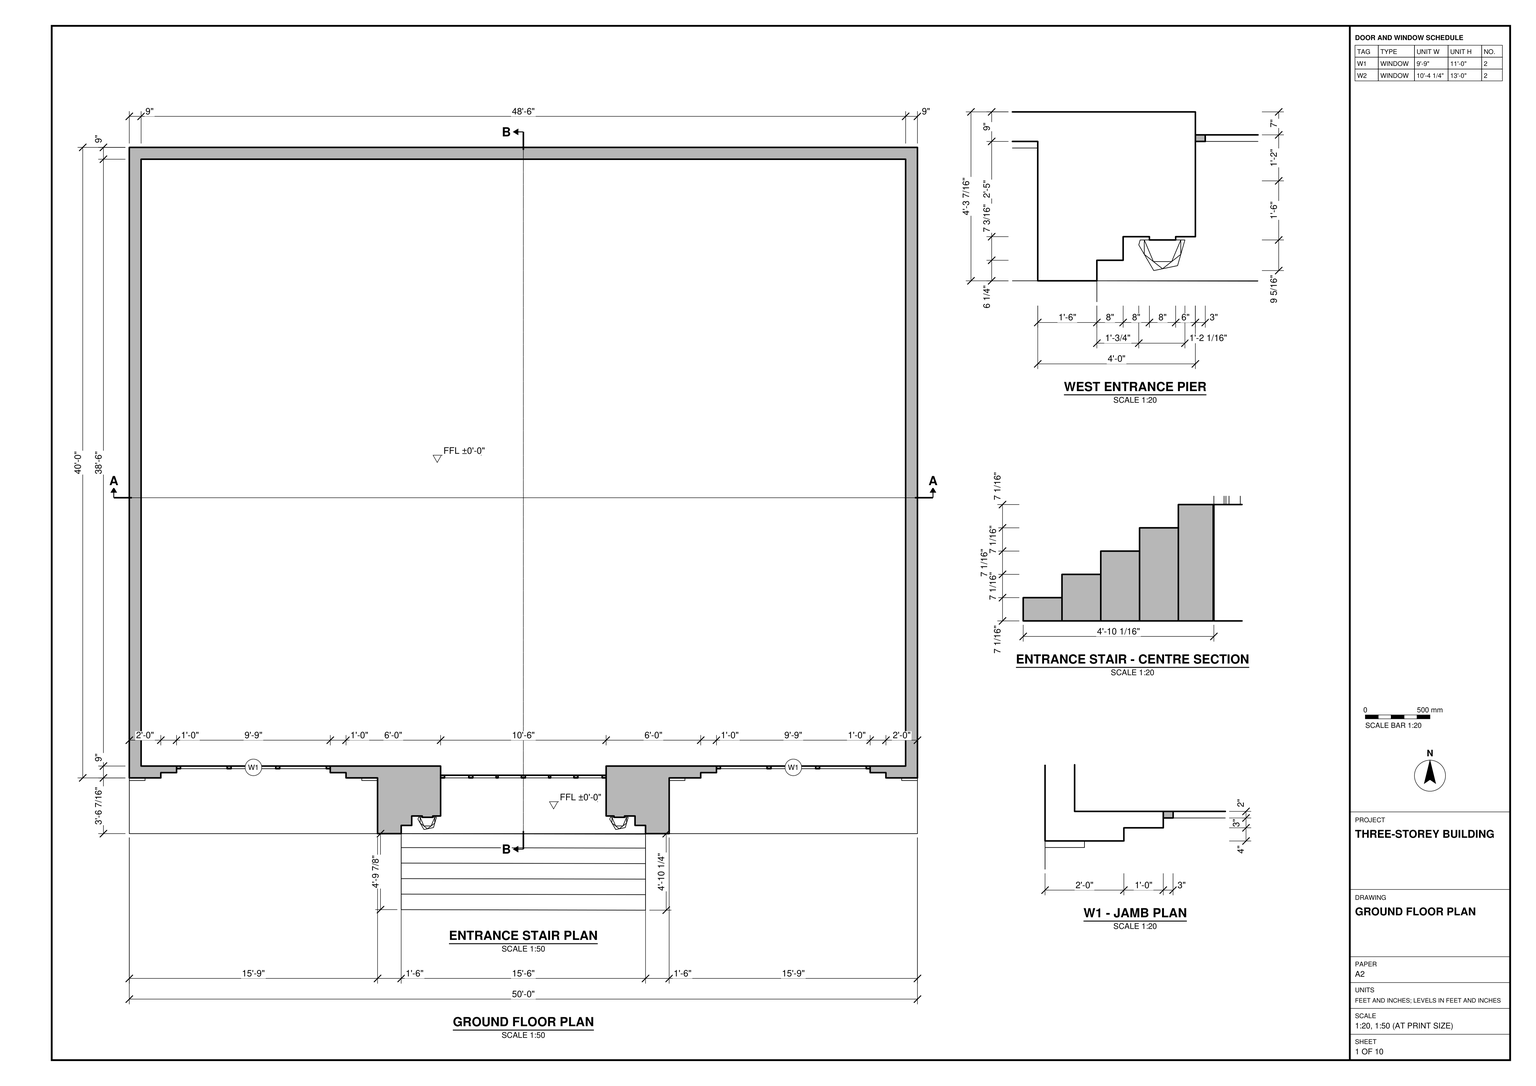
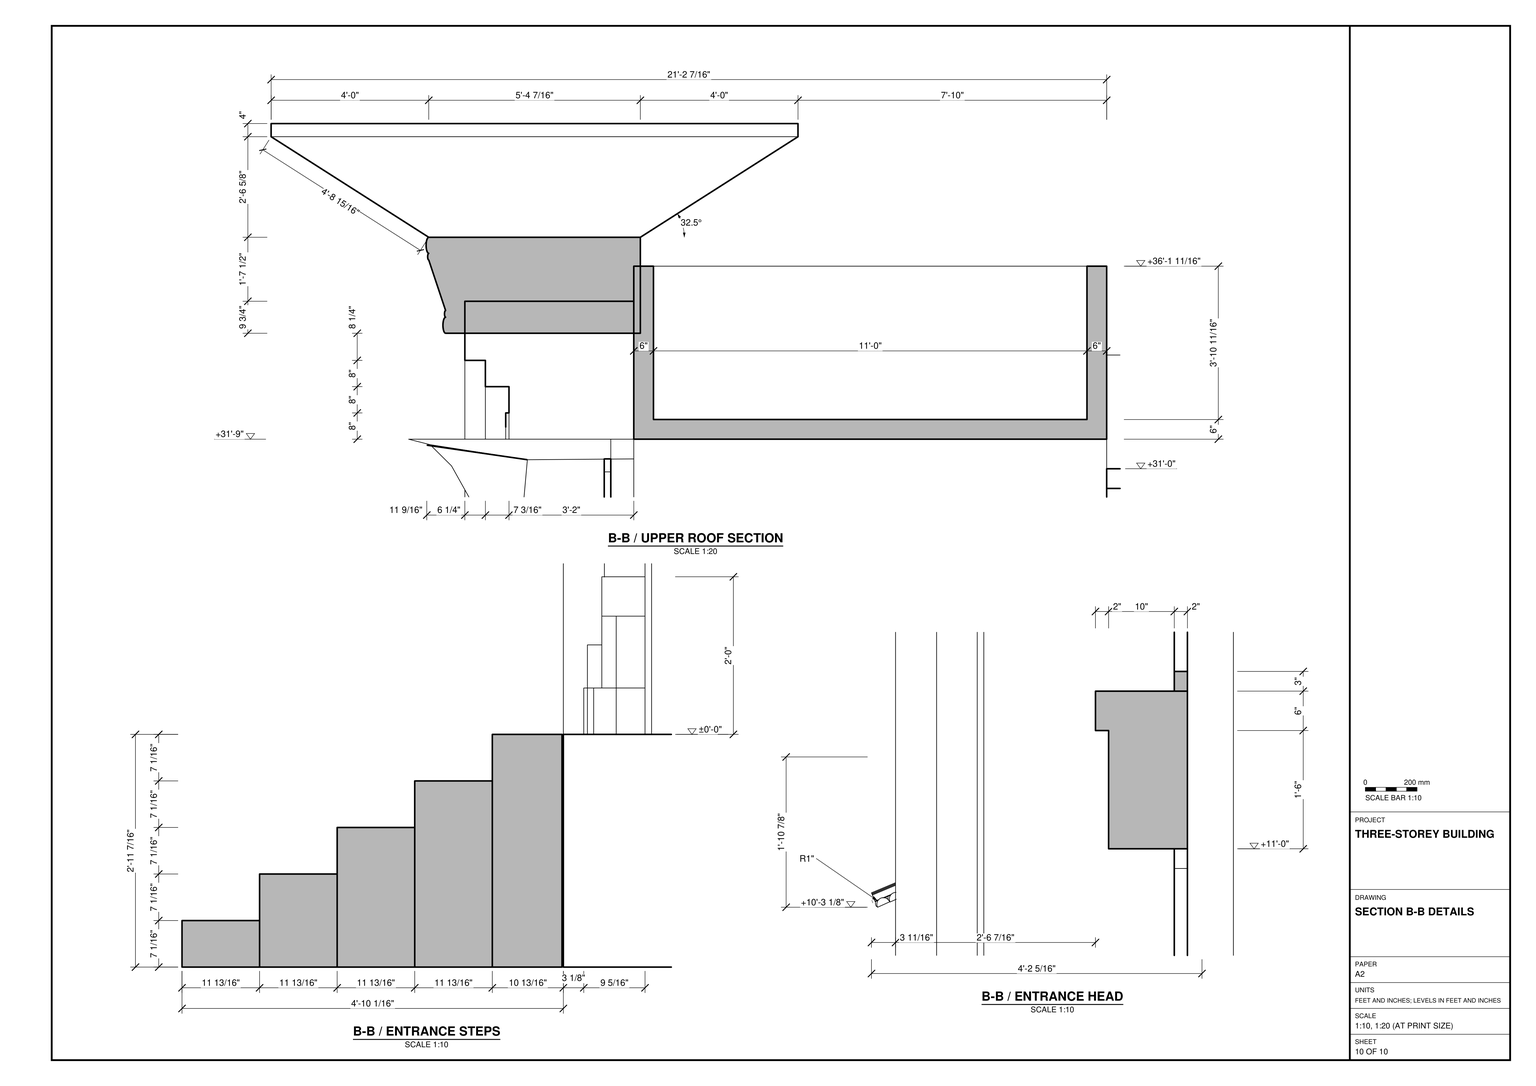
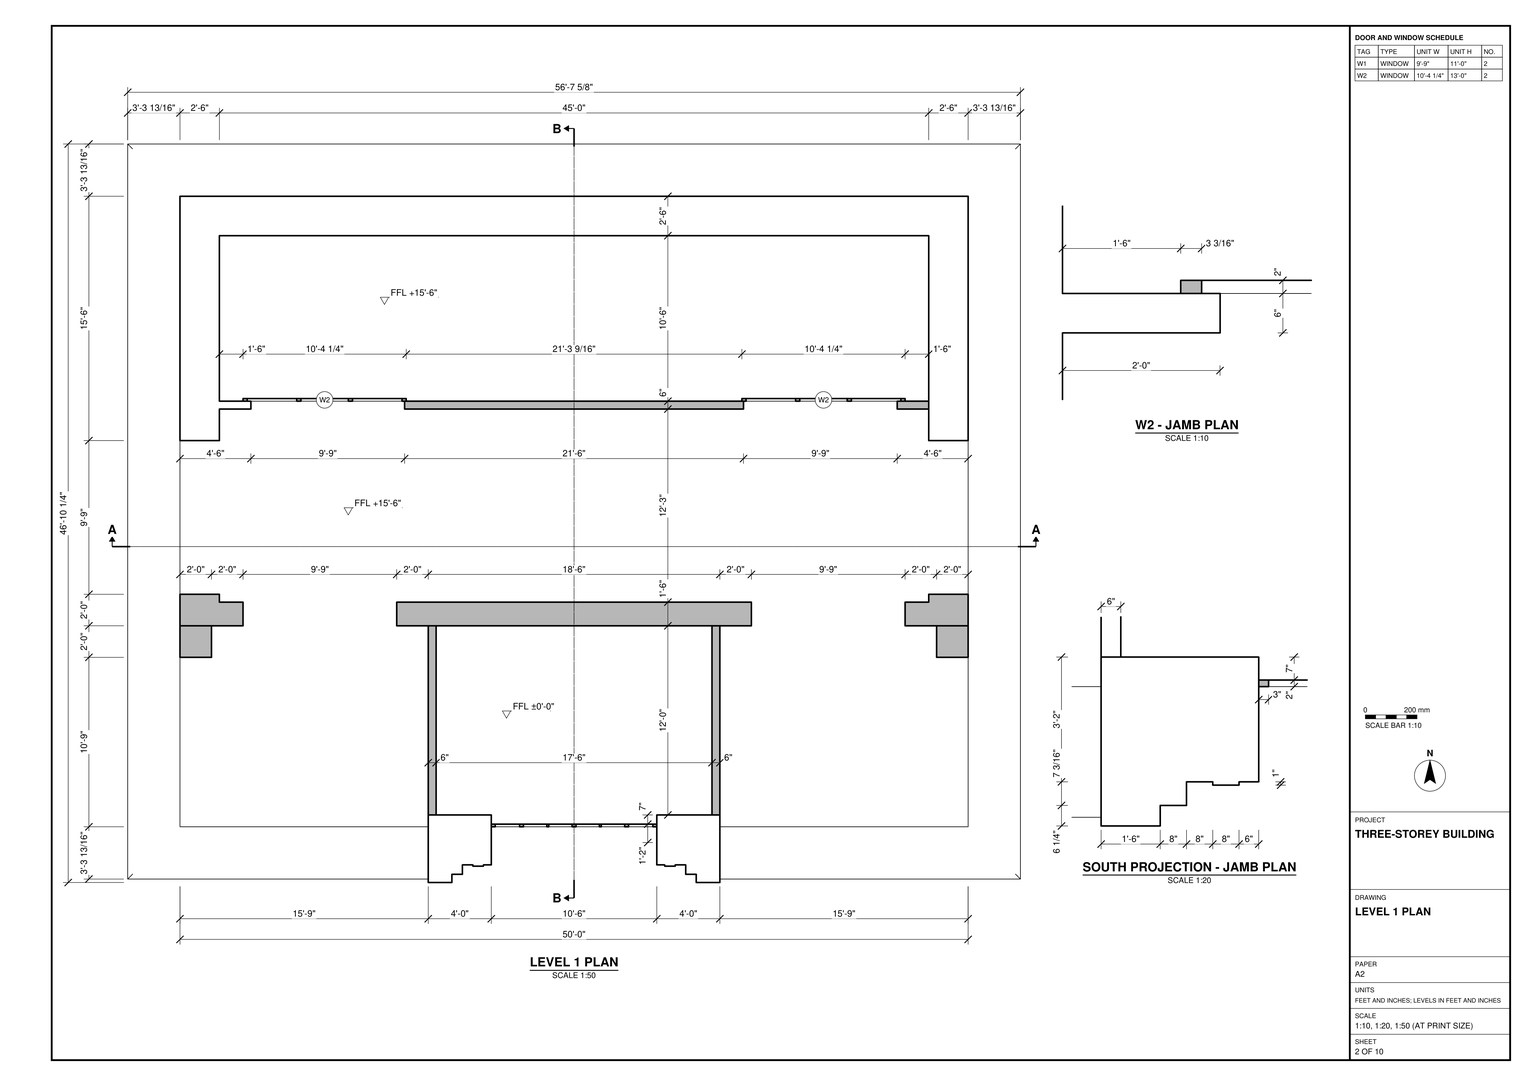
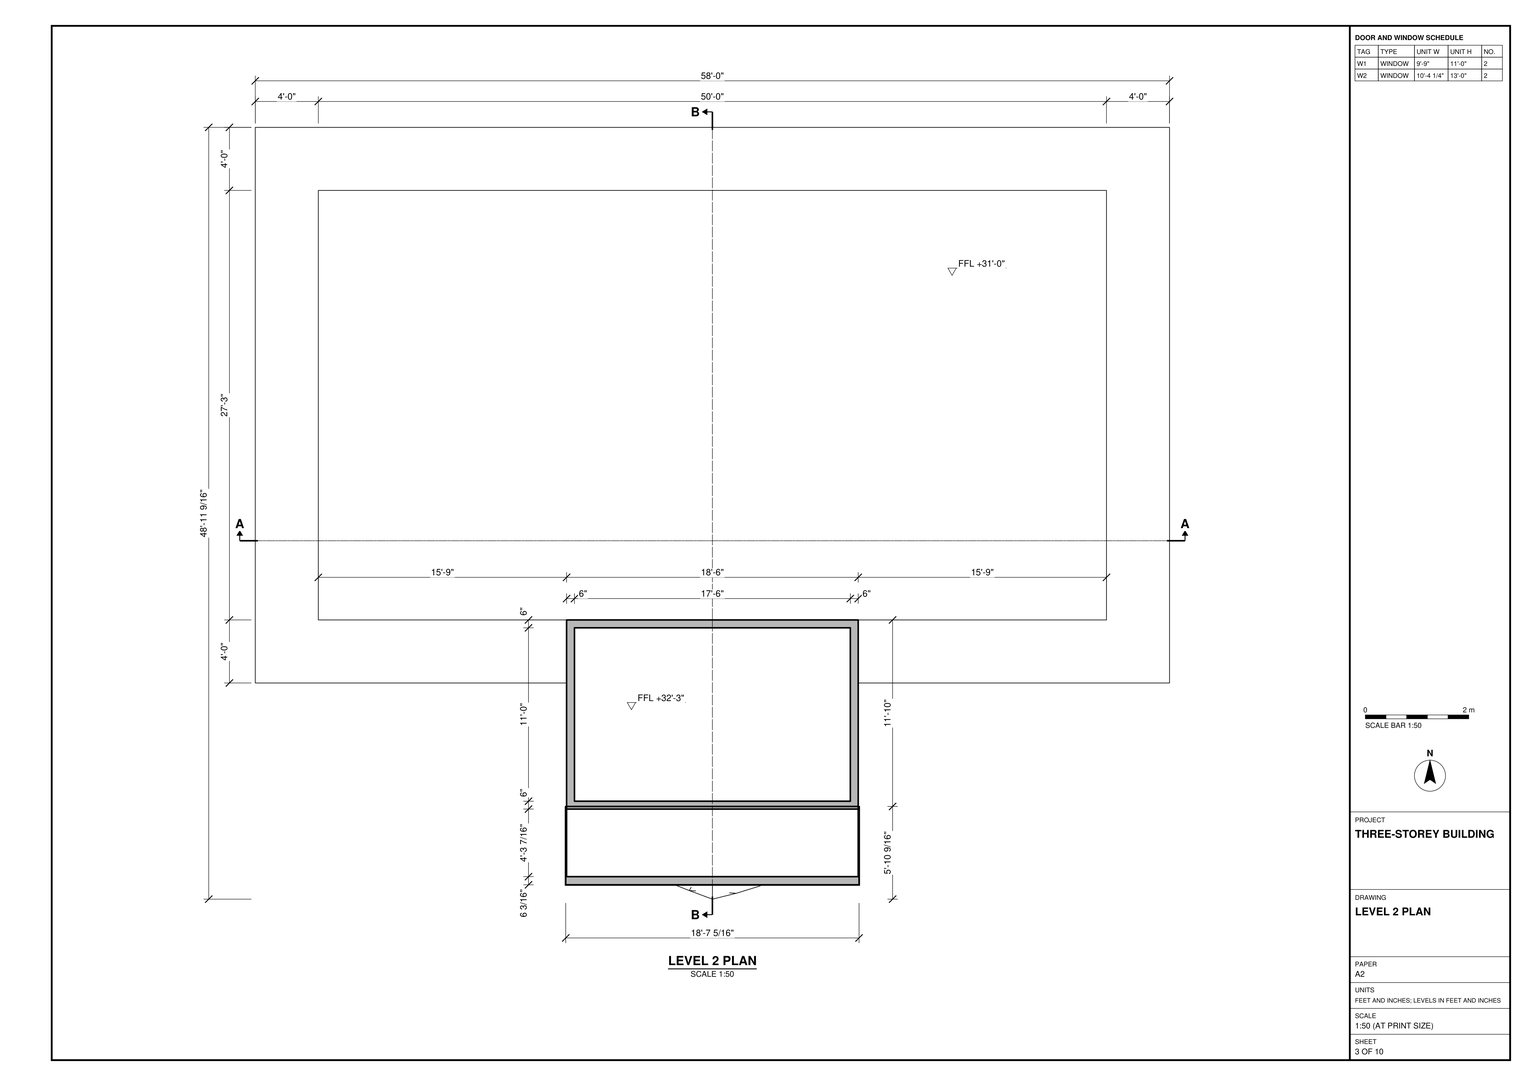
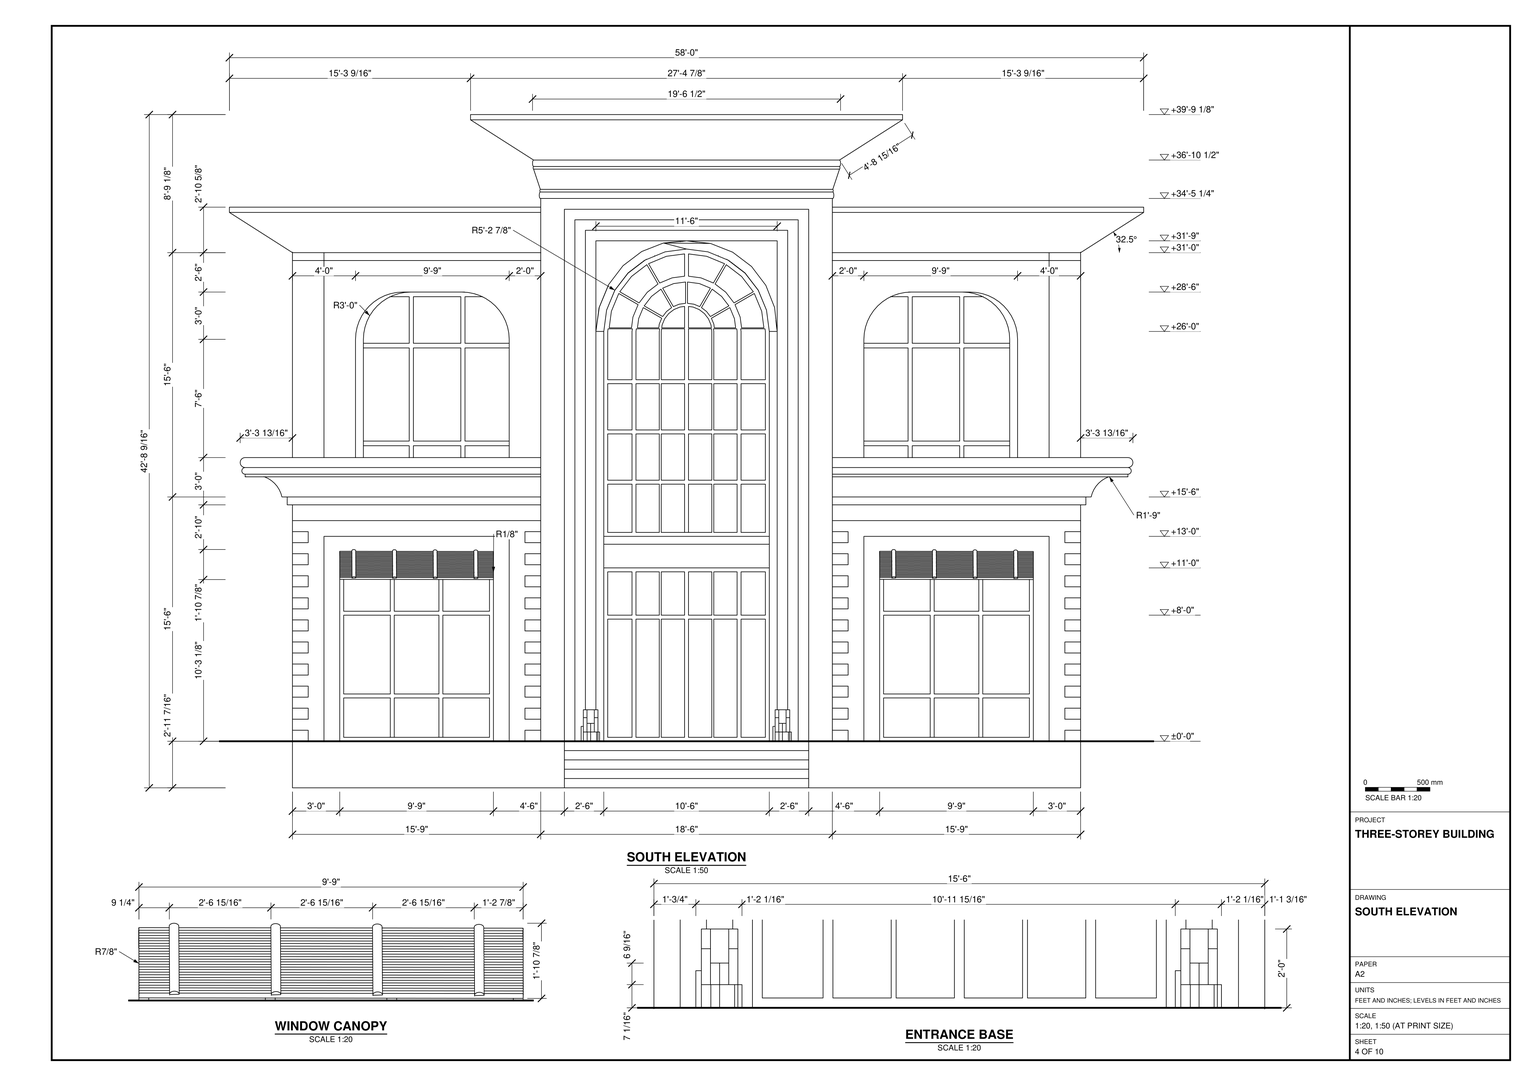
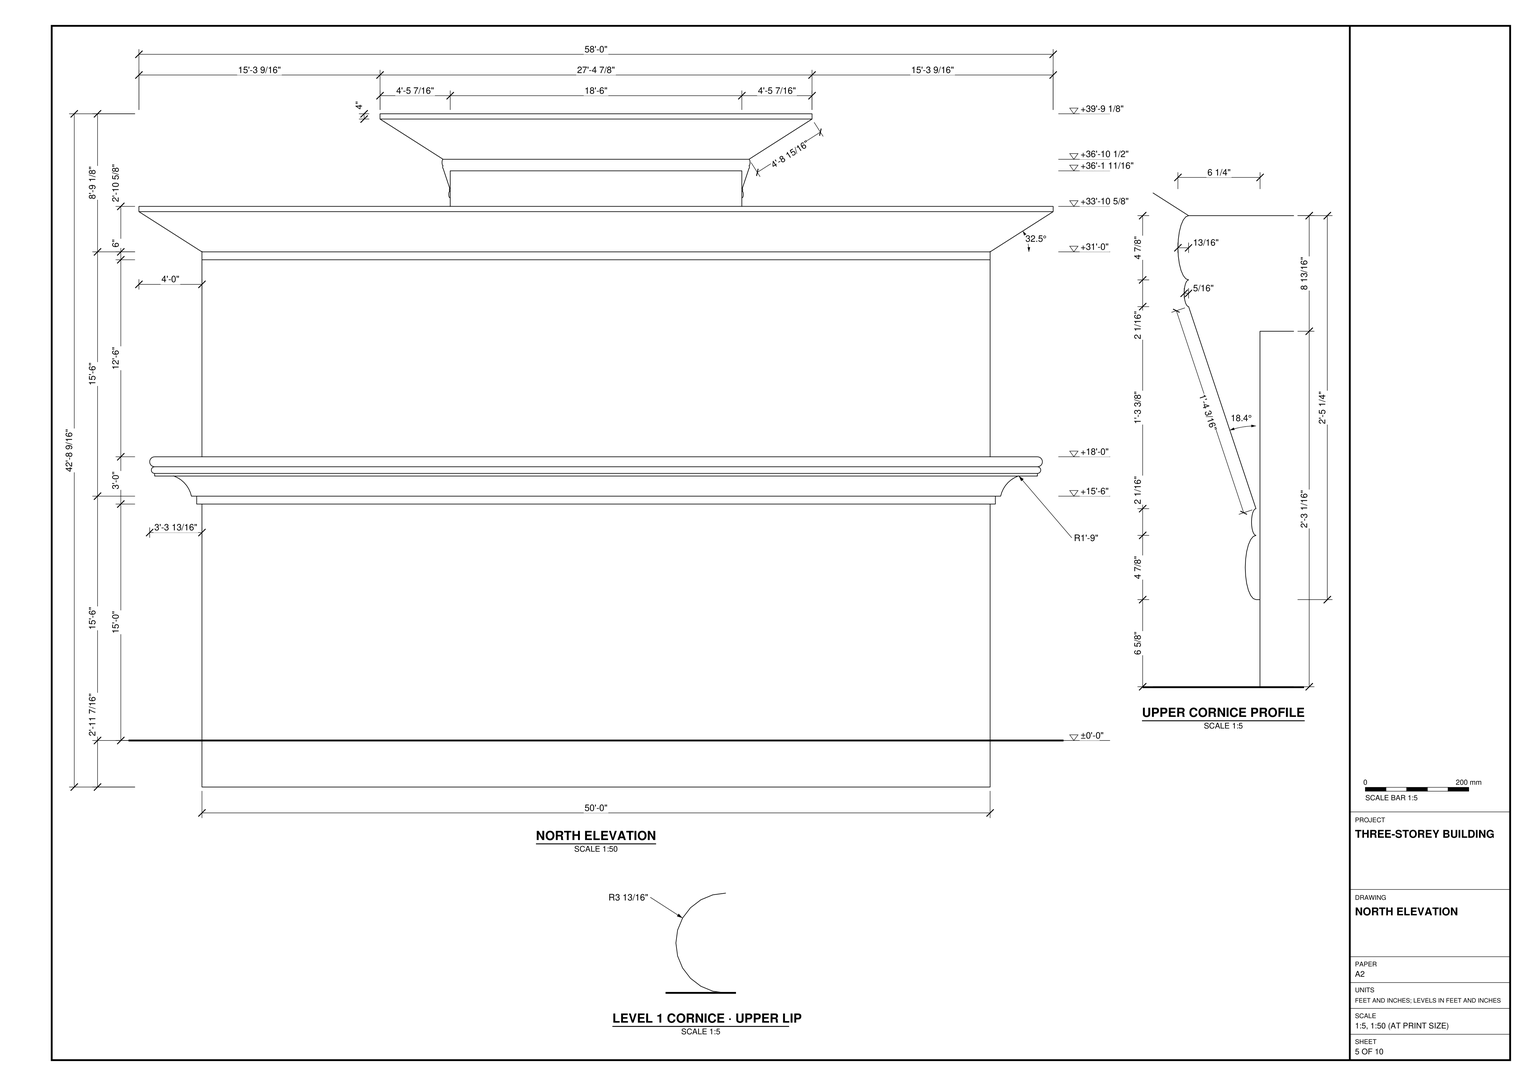
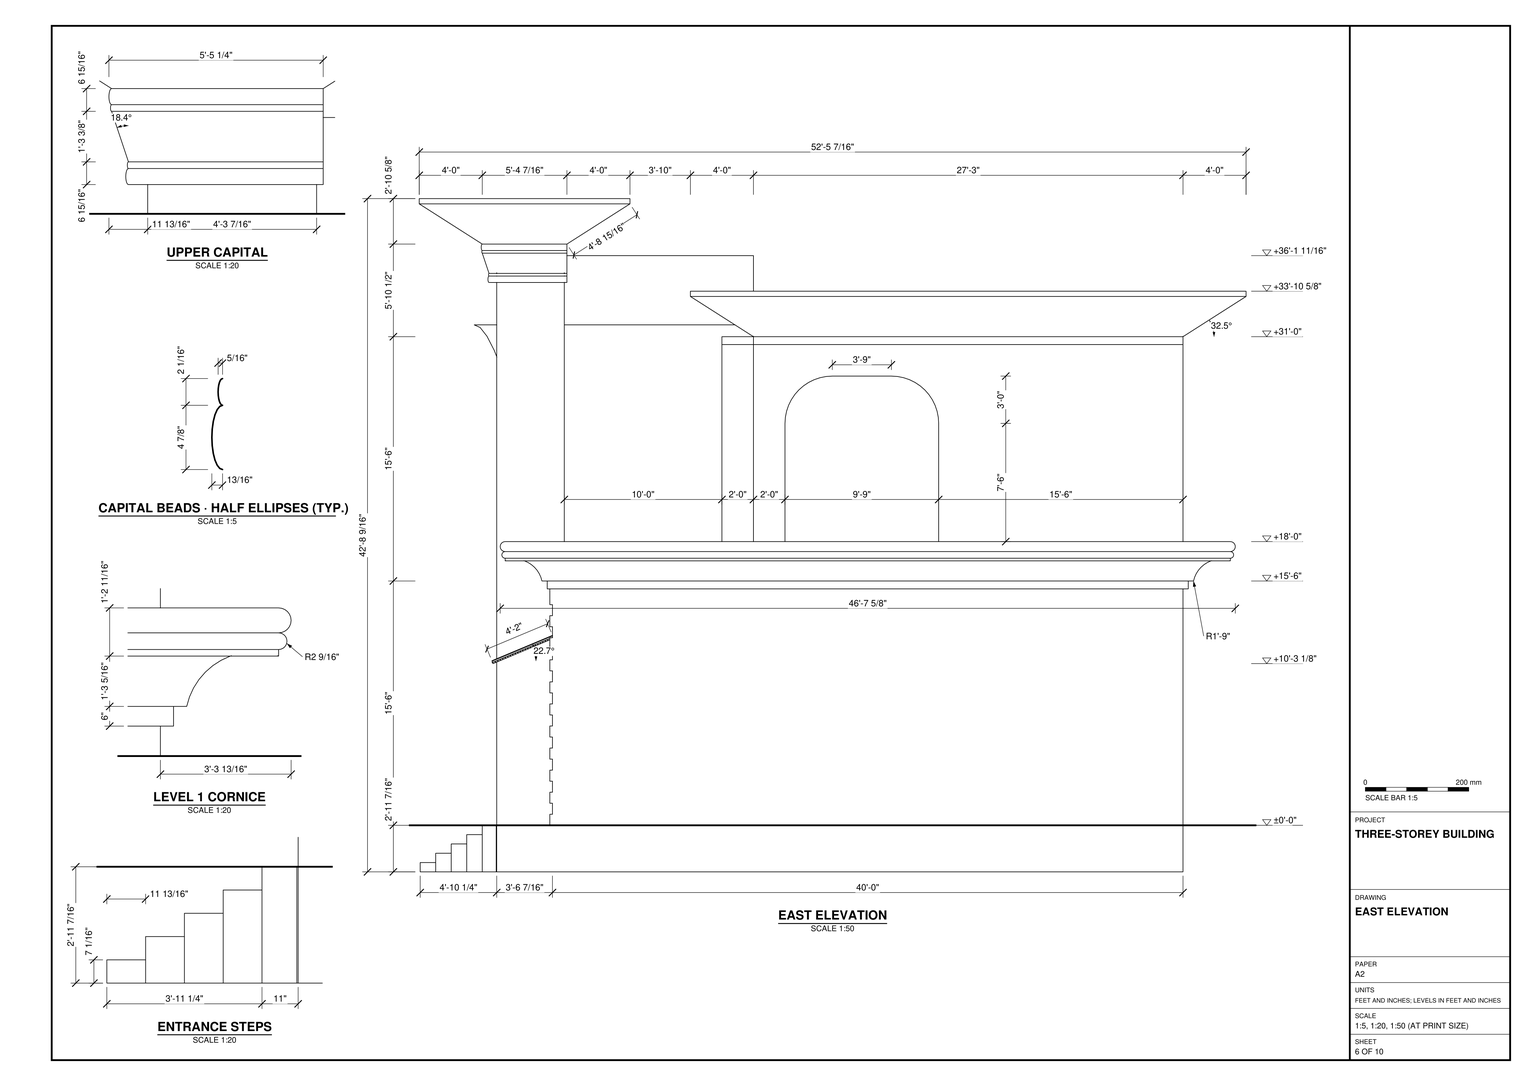
Build the three-storey building in SketchUp from task_files/diagram_01.pdf. Work in feet and inches. The complete model, including its projections, must measure 58'-0" along X, 52'-5 7/16" along Y and 42'-8 9/16" in height. Set the floor levels at ±0'-0", +15'-6" and +31'-0".

Lay out the 50'-0" by 40'-0" ground-floor shell before adding the entrance and roof projections. Model the floor slabs and follow the wall thicknesses in plan, including the 9" side and rear walls at ground level. Centre the entrance on the south face, with a broad flight of steps rising between projecting piers to the entrance opening. Form the stepped jambs and place a tall window on either side of the entrance. At +15'-6", follow the plan setbacks and place the second pair of windows in the south-facing wall of the rear volume. Use the sections to shape the entrance head and the upper roof, including its projecting cap and the adjoining recessed roof area.

Keep walls, slabs and roof elements in separate groups or components, and do the same for each furniture or joinery piece shown. Use components for repeated parts. Any decor or loose items shown may use suitable library components. Save one SketchUp model as output_files/three_storey_building_with_its_stepped_south_entrance.skp.

# SketchUp Ruby script. Lengths in inches.
U = 1.inch
M = Sketchup.active_model
def pt(a) = Geom::Point3d.new(a.map { |v| v * U })
def face(e, loops, mat)
  f = e.add_face(loops[0].map { |a| pt(a) })
  loops[1..].each { |l| e.add_face(l.map { |a| pt(a) }).erase! }
  f.material = f.back_material = mat if mat
  f
end
# faces: each face lists its corners as indices into pts; further lists are holes
def faces(e, pts, list, mat = nil) = list.each { |f| face(e, (f[0].is_a?(Array) ? f : [f]).map { |l| l.map { |i| pts[i] } }, mat) }
# xy, xz, yz: faces in a plane at the given z, y or x. An outline is a flat list of corners, or four numbers for a rectangle; further outlines are holes
def ring(l) = l.size == 4 ? [[l[0], l[1]], [l[2], l[1]], [l[2], l[3]], [l[0], l[3]]] : l.each_slice(2).to_a
def flat(e, list, mat, &to3) = list.each { |f| face(e, (f[0].is_a?(Array) ? f : [f]).map { |l| ring(l).map { |u, v| to3.(u, v) } }, mat) }
def xy(e, z, list, mat = nil) = flat(e, list, mat) { |x, y| [x, y, z] }
def xz(e, y, list, mat = nil) = flat(e, list, mat) { |x, z| [x, y, z] }
def yz(e, x, list, mat = nil) = flat(e, list, mat) { |y, z| [x, y, z] }
def lines(e, pts, list) = list.each { |a, b| e.add_line(pt(pts[a]), pt(pts[b])) }
# prism: a flat outline (further loops are holes) pulled along v
def prism(e, loops, v, mat = nil)
  f = face(e, loops, mat); d = Geom::Vector3d.new(v.map { |x| x * U })
  f.pushpull(f.normal.samedirection?(d) ? d.length : -d.length)
end
def box(e, o, s, mat = nil) = prism(e, [[o, [o[0] + s[0], o[1], o[2]], [o[0] + s[0], o[1] + s[1], o[2]], [o[0], o[1] + s[1], o[2]]]], [0, 0, s[2]], mat)
def at(x, y, z, deg = 0) = Geom::Transformation.translation(pt([x, y, z])) * Geom::Transformation.rotation(ORIGIN, Z_AXIS, deg.degrees)
def axes(o, x, y, z) = Geom::Transformation.new([*x, 0, *y, 0, *z, 0, *pt(o).to_a, 1])
def part(name) = M.definitions.add(name)
# library, detail: a bought-in or finely detailed component or shape, given as its bounding box
def library(name, o, s) = part(name).tap { |d| box(d.entities, o, s) }
def detail(e, o, s) = box(e.add_group.entities, o, s)
def put(e, d, t, mat = nil) = e.add_instance(d, t).tap { |i| i.material = mat if mat }
def group(e, t, mat = nil) = e.add_group.tap { |g| g.transformation = t; g.material = mat if mat }.entities
root = M.entities
M.materials.add("[0034_Wheat]").color = [198, 190, 175]
M.materials.add("[Carrera Marble]").color = [207, 207, 207]
M.materials.add("[Color M06]").color = [86, 86, 86]
M.materials.add("[Color M07]").color = [25, 20, 24]
M.materials.add("[Granite Brown]").color = [126, 104, 91]
M.materials.add("[Tile Veriegated Stone]").color = [171, 137, 112]
M.materials.add("[Translucent Glass Block Dark]").color = [124, 124, 121]
M.materials.add("[Translucent Glass Dark Green]").color = [114, 59, 48]
c1 = part("window")
xy(c1.entities,0,[[0,0,117,2]])
xy(c1.entities,3,[[3,0,38.5,2],[38.5,0,41.5,2],[41.5,0,75.5,2],[75.5,0,78.5,2],[78.5,0,114,2]])
xy(c1.entities,33,[[3,0,38.5,2],[41.5,0,75.5,2],[78.5,0,114,2]])
xy(c1.entities,36,[[3,0,38.5,2],[41.5,0,75.5,2],[78.5,0,114,2]])
xy(c1.entities,96,[[3,0,38.5,2],[41.5,0,75.5,2],[78.5,0,114,2]])
xy(c1.entities,99,[[3,0,38.5,2],[41.5,0,75.5,2],[78.5,0,114,2]])
xy(c1.entities,129,[[3,0,38.5,2],[41.5,0,75.5,2],[78.5,0,114,2]])
xy(c1.entities,132,[[0,0,117,2]])
xz(c1.entities,0,[[[0,0,117,132],[3,3,3,33,38.5,33,38.5,3,41.5,3,41.5,33,75.5,33,75.5,3,78.5,3,78.5,33,114,33,114,3],[3,36,38.5,96],[78.5,36,114,96],[41.5,36,75.5,96],[78.5,99,114,129],[3,99,38.5,129],[41.5,99,75.5,129]]])
xz(c1.entities,2,[[[0,0,117,132],[3,3,114,3,114,33,78.5,33,78.5,3,75.5,3,75.5,33,41.5,33,41.5,3,38.5,3,38.5,33,3,33],[3,36,38.5,96],[78.5,36,114,96],[41.5,36,75.5,96],[78.5,99,114,129],[3,99,38.5,129],[41.5,99,75.5,129]]])
xz(c1.entities,2,[[3,3,38.5,33],[41.5,3,75.5,33],[78.5,3,114,33],[3,36,38.5,96],[41.5,36,75.5,96],
  [78.5,36,114,96],[3,99,38.5,129],[41.5,99,75.5,129],[78.5,99,114,129]],"[Translucent Glass Dark Green]")
yz(c1.entities,0,[[0,0,2,132]])
yz(c1.entities,3,[[0,3,2,33],[0,36,2,96],[0,99,2,129]])
yz(c1.entities,38.5,[[0,3,2,33],[0,36,2,96],[0,99,2,129]])
yz(c1.entities,41.5,[[0,3,2,33],[0,36,2,96],[0,99,2,129]])
yz(c1.entities,75.5,[[0,3,2,33],[0,36,2,96],[0,99,2,129]])
yz(c1.entities,78.5,[[0,3,2,33],[0,36,2,96],[0,99,2,129]])
yz(c1.entities,114,[[0,3,2,33],[0,36,2,96],[0,99,2,129]])
yz(c1.entities,117,[[0,0,2,132]])
c2 = part("Generic Models 17 - Generic Models 17-285328-_3D_")
xy(c2.entities,-17.72,[[-29.13,-33.15,-28.73,33.15,-16.92,33.15,-17.32,-33.15],[-17.32,-33.15,-16.92,33.15,-5.11,33.15,-5.51,-33.15],[-5.51,-33.15,-5.11,33.15,6.7,33.15,6.3,-33.15],[6.3,-33.15,6.7,33.15,18.51,33.15,18.12,-33.15],[18.12,-33.15,18.51,33.15,29.13,33.15,28.73,-33.15]],"[Tile Veriegated Stone]")
xy(c2.entities,-10.63,[[-29.13,-33.15,-17.32,-33.15,-16.92,33.15,-28.73,33.15]],"[Tile Veriegated Stone]")
xy(c2.entities,-3.54,[[-17.32,-33.15,-5.51,-33.15,-5.11,33.15,-16.92,33.15]],"[Tile Veriegated Stone]")
xy(c2.entities,3.54,[[-5.51,-33.15,6.3,-33.15,6.7,33.15,-5.11,33.15]],"[Tile Veriegated Stone]")
xy(c2.entities,10.63,[[6.3,-33.15,18.12,-33.15,18.51,33.15,6.7,33.15]],"[Tile Veriegated Stone]")
xy(c2.entities,17.72,[[18.12,-33.15,28.73,-33.15,29.13,33.15,18.51,33.15]],"[Tile Veriegated Stone]")
xz(c2.entities,-33.15,[[-29.13,-17.72,-17.32,-10.63],[-17.32,-17.72,-5.51,-3.54],[-5.51,-17.72,6.3,3.54],[6.3,-17.72,18.12,10.63],[18.12,-17.72,28.73,17.72]],"[Tile Veriegated Stone]")
xz(c2.entities,33.15,[[-28.73,-17.72,-16.92,-10.63],[-16.92,-17.72,-5.11,-3.54],[-5.11,-17.72,6.7,3.54],[6.7,-17.72,18.51,10.63],[18.51,-17.72,29.13,17.72]],"[Tile Veriegated Stone]")
p = [[-28.73,33.15,-10.63],[-28.73,33.15,-17.72],[-29.13,-33.15,-17.72],[-29.13,-33.15,-10.63],[-16.92,33.15,-3.54],[-16.92,33.15,-17.72],
  [-17.32,-33.15,-17.72],[-17.32,-33.15,-3.54],[-17.32,-33.15,-10.63],[-16.92,33.15,-10.63],[-5.11,33.15,3.54],[-5.11,33.15,-17.72],
  [-5.51,-33.15,-17.72],[-5.51,-33.15,3.54],[-5.51,-33.15,-3.54],[-5.11,33.15,-3.54],[6.7,33.15,10.63],[6.7,33.15,-17.72],
  [6.3,-33.15,-17.72],[6.3,-33.15,10.63],[6.3,-33.15,3.54],[6.7,33.15,3.54],[18.51,33.15,17.72],[18.51,33.15,-17.72],
  [18.12,-33.15,-17.72],[18.12,-33.15,17.72],[18.12,-33.15,10.63],[18.51,33.15,10.63],[28.73,-33.15,17.72],[28.73,-33.15,-17.72],
  [29.13,33.15,-17.72],[29.13,33.15,17.72]]
faces(c2.entities,p,[[0,1,2,3],[4,5,6,7],[8,6,5,9],[10,11,12,13],[14,12,11,15],[16,17,18,19],[20,18,17,21],[22,23,24,25],
  [26,24,23,27],[28,29,30,31]],"[Tile Veriegated Stone]")
c3 = library("Group\#4",[8,99.8125,8],[126,14,375])
c4 = library("Group\#7",[-6.25,-50.07,0],[234.5,65.25,9.74])
c5 = library("Group\#8",[0,-24,0],[600,351,186])
c6 = library("Group\#14",[0,0,0],[679.6,559.6,36])
c7 = part("Component\#1")
xy(c7.entities,0,[[3.83,0.21,5.3,1.0625,6.77,1.91,6.77,3.61,7.43,3.61,6.77,1.91,6.25,0.58]])
xy(c7.entities,7.0625,[[2.42,0,3.83,0.21,2.36,1.0625,0.89,1.91],[3.83,0.21,6.25,0.58,6.77,1.91,7.43,3.61,6.77,3.61,6.77,1.91,5.3,1.0625]])
xy(c7.entities,11.3125,[[0.89,1.91,0.89,3.61,0.23,3.61,0,3.03]])
xy(c7.entities,13.625,[[3.83,0.21,5.3,1.0625,2.36,1.0625]])
xy(c7.entities,18,[[2.36,1.0625,0.89,3.61,0.89,1.91],[5.3,1.0625,6.77,1.91,6.77,3.61]])
xy(c7.entities,24,[[2.36,1.0625,5.3,1.0625,6.77,3.61,0.89,3.61]])
xz(c7.entities,1.0625,[[2.36,13.625,5.3,24]])
xz(c7.entities,3.61,[[0.23,0,0.89,11.3125],[0.89,0,6.77,24],[6.77,0,7.43,7.0625]])
yz(c7.entities,0.89,[[1.91,11.3125,3.61,18]])
yz(c7.entities,6.77,[[1.91,7.0625,3.61,18]])
# 1 loose lines left out
p = [[0.89,1.91,0],[2.42,0,0],[2.42,0,7.0625],[0.89,1.91,7.0625],[3.83,0.21,0],[3.83,0.21,7.0625],
  [6.25,0.58,0],[6.25,0.58,7.0625],[6.77,1.91,0],[6.77,1.91,7.0625],[0,3.03,0],[0.89,1.91,11.3125],
  [0,3.03,11.3125],[7.43,3.61,0],[7.43,3.61,7.0625],[0.23,3.61,0],[0.23,3.61,11.3125],[2.36,1.0625,13.625],
  [2.36,1.0625,7.0625],[3.83,0.21,13.625],[5.3,1.0625,7.0625],[5.3,1.0625,13.625],[2.36,1.0625,18],[0.89,1.91,18],
  [6.77,1.91,18],[5.3,1.0625,18],[0.89,3.61,24],[0.89,3.61,18],[2.36,1.0625,24],[5.3,1.0625,24],
  [6.77,3.61,18],[6.77,3.61,24]]
faces(c7.entities,p,[[0,1,2,3],[1,4,5,2],[4,6,7,5],[6,8,9,7],[10,0,3,11,12],[8,13,14,9],[15,10,12,16],[17,18,5,19],
  [19,5,20,21],[11,3,18,17,22,23],[21,20,9,24,25],[26,27,22,28],[29,25,30,31]])
c8 = library("Group\#57",[0,-0.05,0],[53.97,2.25,80.01])
p = [[237,110.43,204],[237,110.43,210]]
lines(root,p,[[0,1]])
put(root,c1,at(84,108.43,24),"[Color M07]")
put(root,c1,at(495,108.43,24),"[Color M07]")
put(root,c1,axes([475.77,425.43,210],[1.06179,0,0],[0,1,0],[0,0,1.18182]),"[Color M07]")
put(root,c1,axes([96,425.43,210],[1.06179,0,0],[0,1,0],[0,0,1.18182]),"[Color M07]")
put(root,c2,axes([348,29.87,6.28],[0,1,0],[-2.8057,0,0],[0,0,1]),"[Tile Veriegated Stone]")
g1 = group(root,at(48,-18.57,0),"[Tile Veriegated Stone]")
xy(g1,-11.43,[[0,77.5625,600,600]])
xy(g1,24,[[0,77.5625,600,600]],"[Granite Brown]")
xz(g1,77.5625,[[0,-11.43,600,24]])
xz(g1,600,[[0,-11.43,600,24]])
yz(g1,0,[[77.5625,-11.43,600,24]])
yz(g1,600,[[77.5625,-11.43,600,24]])
g2 = group(root,at(48,101.43,204),"[0034_Wheat]")
xy(g2,0,[[0,0,0,480,600,480,600,0,411,0,411,153,189,153,189,0],[189,9,195,153],[405,9,411,153]])
xy(g2,6,[[0,0,189,0,189,153,411,153,411,0,600,0,600,480,0,480]],"[Carrera Marble]")
xy(g2,201,[[189,9,195,153],[405,9,411,153]])
xz(g2,0,[[0,0,189,6],[411,0,600,6]])
xz(g2,9,[[189,0,195,201],[405,0,411,201]])
xz(g2,153,[[189,0,195,6],[195,0,405,6],[405,0,411,6],[189,6,195,201],[405,6,411,201]])
xz(g2,480,[[0,0,600,6]])
yz(g2,0,[[0,0,480,6]])
yz(g2,189,[[0,0,9,6],[9,0,153,6],[9,6,153,201]])
yz(g2,195,[[9,0,153,201]])
yz(g2,405,[[9,0,153,201]])
yz(g2,411,[[0,0,9,6],[9,0,153,6],[9,6,153,201]])
yz(g2,600,[[0,0,480,6]])
put(root,c3,at(277,-10.38,16),"[Color M07]")
put(root,c4,axes([237,97.25,437.26],[1,0,0],[0,1,0],[0,0,3]),"[0034_Wheat]")
put(root,c5,at(48,254.43,210),"[0034_Wheat]")
g3 = group(root,at(48,254.43,390),"[0034_Wheat]")
box(g3,[0,0,0],[600,327,6])
g4 = group(root,at(48,254.43,396),"[Color M06]")
xy(g4,34.625,[[-48,-48,189,-48,189,0,0,0,0,327,600,327,600,0,411,0,411,-48,648,-48,648,375,-48,375]])
xz(g4,-48,[[-48,30.625,189,34.625],[411,30.625,648,34.625]])
xz(g4,0,[[0,0,189,34.625],[411,0,600,34.625]])
xz(g4,327,[[0,0,600,34.625]])
xz(g4,375,[[-48,30.625,648,34.625]])
yz(g4,-48,[[-48,30.625,375,34.625]])
yz(g4,0,[[0,0,327,34.625]])
yz(g4,189,[[0,0,0,34.625,-48,34.625,-48,30.625]])
yz(g4,411,[[0,0,-48,30.625,-48,34.625,0,34.625]])
yz(g4,600,[[0,0,327,34.625]])
yz(g4,648,[[-48,30.625,375,34.625]])
p = [[-48,375,30.625],[0,327,0],[0,0,0],[-48,-48,30.625],[189,0,0],[189,-48,30.625],
  [600,0,0],[648,-48,30.625],[411,-48,30.625],[411,0,0],[600,327,0],[648,375,30.625]]
faces(g4,p,[[0,1,2,3],[3,2,4,5],[6,7,8,9],[10,11,7,6],[11,10,1,0]])
g5 = group(root,at(237,110.43,405),"[Color M06]")
xy(g5,0,[[0,0,222,144]])
xy(g5,6,[[6,6,216,138]])
xy(g5,52.6875,[[[0,0,222,144],[6,6,216,138]]])
xz(g5,0,[[0,0,222,52.6875]])
xz(g5,6,[[6,6,216,52.6875]])
xz(g5,138,[[6,6,216,52.6875]])
xz(g5,144,[[0,0,222,52.6875]])
yz(g5,0,[[0,0,144,52.6875]])
yz(g5,6,[[6,6,138,52.6875]])
yz(g5,216,[[6,6,138,52.6875]])
yz(g5,222,[[0,0,144,52.6875]])
g6 = group(root,at(183.57,0,466.49),"[Color M06]")
xy(g6,0,[[48,48,280.86,112.43]])
xy(g6,34.625,[[0,0,328.86,160.43]])
xz(g6,0,[[0,30.625,328.86,34.625]])
xz(g6,160.43,[[0,30.625,328.86,34.625]])
yz(g6,0,[[0,30.625,160.43,34.625]])
yz(g6,328.86,[[0,30.625,160.43,34.625]])
p = [[48,48,0],[0,0,30.625],[0,160.43,30.625],[48,112.43,0],[280.86,48,0],[328.86,0,30.625],
  [280.86,112.43,0],[328.86,160.43,30.625]]
faces(g6,p,[[0,1,2,3],[4,5,1,0],[6,7,5,4],[3,2,7,6]])
put(root,c6,at(8.2,61.63,204),"[0034_Wheat]")
g7 = group(root,at(48,101.43,24),"[0034_Wheat]")
xy(g7,0,[[189,-42.4375,189,-2,177,-2,177,0,165,0,165,4,153,4,153,9,237,9,237,-29,231,-29,231,-30,223,-30,223,-29,215,-29,215,-36.1875,207,-36.1875,207,-42.4375],[393,-42.4375,393,-36.1875,385,-36.1875,385,-29,377,-29,377,-30,369,-30,369,-29,363,-29,363,9,447,9,447,4,435,4,435,0,423,0,423,-2,411,-2,411,-42.4375],[0,-2,0,480,600,480,600,-2,588,-2,588,0,576,0,576,4,564,4,564,9,591,9,591,471,9,471,9,9,36,9,36,4,24,4,24,0,12,0,12,-2]])
xy(g7,8.4,[[0,-2,12,0],[177,-2,189,0],[411,-2,423,0],[588,-2,600,0]])
xy(g7,16.8,[[0,-2,12,0],[177,-2,189,0],[411,-2,423,0],[588,-2,600,0]])
xy(g7,25.2,[[0,-2,12,0],[177,-2,189,0],[411,-2,423,0],[588,-2,600,0]])
xy(g7,33.6,[[0,-2,12,0],[177,-2,189,0],[411,-2,423,0],[588,-2,600,0]])
xy(g7,42,[[0,-2,12,0],[177,-2,189,0],[411,-2,423,0],[588,-2,600,0]])
xy(g7,50.4,[[0,-2,12,0],[177,-2,189,0],[411,-2,423,0],[588,-2,600,0]])
xy(g7,58.8,[[0,-2,12,0],[177,-2,189,0],[411,-2,423,0],[588,-2,600,0]])
xy(g7,67.2,[[0,-2,12,0],[177,-2,189,0],[411,-2,423,0],[588,-2,600,0]])
xy(g7,75.6,[[0,-2,12,0],[177,-2,189,0],[411,-2,423,0],[588,-2,600,0]])
xy(g7,84,[[0,-2,12,0],[177,-2,189,0],[411,-2,423,0],[588,-2,600,0]])
xy(g7,92.4,[[0,-2,12,0],[177,-2,189,0],[411,-2,423,0],[588,-2,600,0]])
xy(g7,100.8,[[0,-2,12,0],[177,-2,189,0],[411,-2,423,0],[588,-2,600,0]])
xy(g7,109.2,[[0,-2,12,0],[177,-2,189,0],[411,-2,423,0],[588,-2,600,0]])
xy(g7,117.6,[[0,-2,12,0],[177,-2,189,0],[411,-2,423,0],[588,-2,600,0]])
xy(g7,126,[[0,-2,12,0],[177,-2,189,0],[411,-2,423,0],[588,-2,600,0]])
xy(g7,134.4,[[0,-2,12,0],[177,-2,189,0],[411,-2,423,0],[588,-2,600,0]])
xy(g7,142.8,[[0,-2,12,0],[177,-2,189,0],[411,-2,423,0],[588,-2,600,0]])
xy(g7,144,[[36,4,153,9],[447,4,564,9]])
xy(g7,151.2,[[0,-2,12,0],[177,-2,189,0],[411,-2,423,0],[588,-2,600,0]])
xy(g7,156,[[24,0,165,4],[435,0,576,4]])
xy(g7,159.6,[[0,-2,12,0],[177,-2,189,0],[411,-2,423,0],[588,-2,600,0]])
xy(g7,168,[[0,-2,189,0],[411,-2,600,0]])
xy(g7,180,[[0,-2,189,-2,189,9,9,9,9,471,591,471,591,9,411,9,411,-2,600,-2,600,480,0,480]])
xy(g7,381,[[231,-30,300,9],[300,-30,366.65,9],[366.65,-30,369,9]])
xy(g7,389,[[223,-30,377,-29]])
xy(g7,397,[[215,-36.1875,385,-29]])
xy(g7,405,[[207,-42.4375,393,-36.1875]])
xy(g7,423,[[189,-42.4375,411,9]])
xz(g7,-42.4375,[[189,0,207,0,207,405,393,405,393,0,411,0,411,423,189,423]])
xz(g7,-36.1875,[[207,0,215,0,215,397,385,397,385,0,393,0,393,405,207,405]])
xz(g7,-30,[[223,0,231,0,231,381,369,381,369,0,377,0,377,389,223,389]])
xz(g7,-29,[[215,0,223,0,223,389,377,389,377,0,385,0,385,397,215,397],[231,0,237,312],[363,0,369,312]])
xz(g7,-2,[[0,0,12,8.4],[177,0,189,8.4],[411,0,423,8.4],[588,0,600,8.4],[0,16.8,12,25.2],
  [177,16.8,189,25.2],[411,16.8,423,25.2],[588,16.8,600,25.2],[0,33.6,12,42],[177,33.6,189,42],
  [411,33.6,423,42],[588,33.6,600,42],[0,50.4,12,58.8],[177,50.4,189,58.8],[411,50.4,423,58.8],
  [588,50.4,600,58.8],[0,67.2,12,75.6],[177,67.2,189,75.6],[411,67.2,423,75.6],[588,67.2,600,75.6],
  [0,84,12,92.4],[177,84,189,92.4],[411,84,423,92.4],[588,84,600,92.4],[0,100.8,12,109.2],
  [177,100.8,189,109.2],[411,100.8,423,109.2],[588,100.8,600,109.2],[0,117.6,12,126],[177,117.6,189,126],
  [411,117.6,423,126],[588,117.6,600,126],[0,134.4,12,142.8],[177,134.4,189,142.8],[411,134.4,423,142.8],
  [588,134.4,600,142.8],[0,151.2,12,159.6],[177,151.2,189,159.6],[411,151.2,423,159.6],[588,151.2,600,159.6],
  [0,168,189,180],[411,168,600,180]])
xz(g7,0,[[12,0,24,0,24,156,165,156,165,0,177,0,177,8.4,189,8.4,189,16.8,177,16.8,177,25.2,189,25.2,189,33.6,177,33.6,177,42,189,42,189,50.4,177,50.4,177,58.8,189,58.8,189,67.2,177,67.2,177,75.6,189,75.6,189,84,177,84,177,92.4,189,92.4,189,100.8,177,100.8,177,109.2,189,109.2,189,117.6,177,117.6,177,126,189,126,189,134.4,177,134.4,177,142.8,189,142.8,189,151.2,177,151.2,177,159.6,189,159.6,189,168,0,168,0,159.6,12,159.6,12,151.2,0,151.2,0,142.8,12,142.8,12,134.4,0,134.4,0,126,12,126,12,117.6,0,117.6,0,109.2,12,109.2,12,100.8,0,100.8,0,92.4,12,92.4,12,84,0,84,0,75.6,12,75.6,12,67.2,0,67.2,0,58.8,12,58.8,12,50.4,0,50.4,0,42,12,42,12,33.6,0,33.6,0,25.2,12,25.2,12,16.8,0,16.8,0,8.4,12,8.4],[423,0,435,0,435,156,576,156,576,0,588,0,588,8.4,600,8.4,600,16.8,588,16.8,588,25.2,600,25.2,600,33.6,588,33.6,588,42,600,42,600,50.4,588,50.4,588,58.8,600,58.8,600,67.2,588,67.2,588,75.6,600,75.6,600,84,588,84,588,92.4,600,92.4,600,100.8,588,100.8,588,109.2,600,109.2,600,117.6,588,117.6,588,126,600,126,600,134.4,588,134.4,588,142.8,600,142.8,600,151.2,588,151.2,588,159.6,600,159.6,600,168,411,168,411,159.6,423,159.6,423,151.2,411,151.2,411,142.8,423,142.8,423,134.4,411,134.4,411,126,423,126,423,117.6,411,117.6,411,109.2,423,109.2,423,100.8,411,100.8,411,92.4,423,92.4,423,84,411,84,411,75.6,423,75.6,423,67.2,411,67.2,411,58.8,423,58.8,423,50.4,411,50.4,411,42,423,42,423,33.6,411,33.6,411,25.2,423,25.2,423,16.8,411,16.8,411,8.4,423,8.4]])
xz(g7,4,[[24,0,36,0,36,144,153,144,153,0,165,0,165,156,24,156],[435,0,447,0,447,144,564,144,564,0,576,0,576,156,435,156]])
xz(g7,9,[[[9,0,9,180,189,180,189,423,411,423,411,180,591,180,591,0,564,0,564,144,447,144,447,0,363,0,363,312,360.85,328.31,354.56,343.5,344.55,356.55,331.5,366.56,316.31,372.85,300,375,283.69,372.85,268.5,366.56,255.45,356.55,245.44,343.5,239.15,328.31,237,312,237,0,153,0,153,144,36,144,36,0],[369,312,369,381,300,381,317.86,378.65,334.5,371.76,348.79,360.79,359.76,346.5,366.65,329.86],[231,312,233.35,329.86,240.24,346.5,251.21,360.79,265.5,371.76,282.14,378.65,300,381,231,381]]])
xz(g7,471,[[9,0,591,180]])
xz(g7,480,[[0,0,600,180]])
yz(g7,0,[[-2,0,-2,8.4,0,8.4,0,16.8,-2,16.8,-2,25.2,0,25.2,0,33.6,-2,33.6,-2,42,0,42,0,50.4,-2,50.4,-2,58.8,0,58.8,0,67.2,-2,67.2,-2,75.6,0,75.6,0,84,-2,84,-2,92.4,0,92.4,0,100.8,-2,100.8,-2,109.2,0,109.2,0,117.6,-2,117.6,-2,126,0,126,0,134.4,-2,134.4,-2,142.8,0,142.8,0,151.2,-2,151.2,-2,159.6,0,159.6,0,168,-2,168,-2,180,480,180,480,0]])
yz(g7,9,[[9,0,471,180]])
yz(g7,12,[[-2,0,0,8.4],[-2,16.8,0,25.2],[-2,33.6,0,42],[-2,50.4,0,58.8],[-2,67.2,0,75.6],
  [-2,84,0,92.4],[-2,100.8,0,109.2],[-2,117.6,0,126],[-2,134.4,0,142.8],[-2,151.2,0,159.6]])
yz(g7,24,[[0,0,4,156]])
yz(g7,36,[[4,0,9,144]])
yz(g7,153,[[4,0,9,144]])
yz(g7,165,[[0,0,4,156]])
yz(g7,177,[[-2,0,0,8.4],[-2,16.8,0,25.2],[-2,33.6,0,42],[-2,50.4,0,58.8],[-2,67.2,0,75.6],
  [-2,84,0,92.4],[-2,100.8,0,109.2],[-2,117.6,0,126],[-2,134.4,0,142.8],[-2,151.2,0,159.6]])
yz(g7,189,[[-42.4375,0,-42.4375,423,9,423,9,180,-2,180,-2,168,0,168,0,159.6,-2,159.6,-2,151.2,0,151.2,0,142.8,-2,142.8,-2,134.4,0,134.4,0,126,-2,126,-2,117.6,0,117.6,0,109.2,-2,109.2,-2,100.8,0,100.8,0,92.4,-2,92.4,-2,84,0,84,0,75.6,-2,75.6,-2,67.2,0,67.2,0,58.8,-2,58.8,-2,50.4,0,50.4,0,42,-2,42,-2,33.6,0,33.6,0,25.2,-2,25.2,-2,16.8,0,16.8,0,8.4,-2,8.4,-2,0]])
yz(g7,207,[[-42.4375,0,-36.1875,405]])
yz(g7,215,[[-36.1875,0,-29,397]])
yz(g7,223,[[-30,0,-29,389]])
yz(g7,231,[[-30,0,-29,0,-29,312,9,312,9,381,-30,381]])
yz(g7,237,[[-29,0,9,312]])
yz(g7,363,[[-29,0,9,312]])
yz(g7,369,[[-30,0,-29,312],[-30,312,9,381]])
yz(g7,377,[[-30,0,-29,389]])
yz(g7,385,[[-36.1875,0,-29,397]])
yz(g7,393,[[-42.4375,0,-36.1875,405]])
yz(g7,411,[[-42.4375,0,-2,0,-2,8.4,0,8.4,0,16.8,-2,16.8,-2,25.2,0,25.2,0,33.6,-2,33.6,-2,42,0,42,0,50.4,-2,50.4,-2,58.8,0,58.8,0,67.2,-2,67.2,-2,75.6,0,75.6,0,84,-2,84,-2,92.4,0,92.4,0,100.8,-2,100.8,-2,109.2,0,109.2,0,117.6,-2,117.6,-2,126,0,126,0,134.4,-2,134.4,-2,142.8,0,142.8,0,151.2,-2,151.2,-2,159.6,0,159.6,0,168,-2,168,-2,180,9,180,9,423,-42.4375,423]])
yz(g7,423,[[-2,0,0,8.4],[-2,16.8,0,25.2],[-2,33.6,0,42],[-2,50.4,0,58.8],[-2,67.2,0,75.6],
  [-2,84,0,92.4],[-2,100.8,0,109.2],[-2,117.6,0,126],[-2,134.4,0,142.8],[-2,151.2,0,159.6]])
yz(g7,435,[[0,0,4,156]])
yz(g7,447,[[4,0,9,144]])
yz(g7,564,[[4,0,9,144]])
yz(g7,576,[[0,0,4,156]])
yz(g7,588,[[-2,0,0,8.4],[-2,16.8,0,25.2],[-2,33.6,0,42],[-2,50.4,0,58.8],[-2,67.2,0,75.6],
  [-2,84,0,92.4],[-2,100.8,0,109.2],[-2,117.6,0,126],[-2,134.4,0,142.8],[-2,151.2,0,159.6]])
yz(g7,591,[[9,0,471,180]])
yz(g7,600,[[-2,0,480,0,480,180,-2,180,-2,168,0,168,0,159.6,-2,159.6,-2,151.2,0,151.2,0,142.8,-2,142.8,-2,134.4,0,134.4,0,126,-2,126,-2,117.6,0,117.6,0,109.2,-2,109.2,-2,100.8,0,100.8,0,92.4,-2,92.4,-2,84,0,84,0,75.6,-2,75.6,-2,67.2,0,67.2,0,58.8,-2,58.8,-2,50.4,0,50.4,0,42,-2,42,-2,33.6,0,33.6,0,25.2,-2,25.2,-2,16.8,0,16.8,0,8.4,-2,8.4]])
p = [[360.85,-27.55,328.24],[363,-29,312],[367.02,-33.48,330.23],[369,-29,312],[366.65,0,329.86],[233.59,-31.4,330.54],
  [233.35,2,329.86],[231,-29,312],[239.15,-27.55,328.24],[237,-29,312],[231,2,312],[239.15,9,328.31],
  [237,9,312],[360.85,9,328.31],[363,9,312],[369,0,312],[369,9,312],[366.65,9,329.86],
  [233.35,9,329.86],[231,9,312],[354.56,-26.2,343.375],[245.44,-26.2,343.375],[354.56,9,343.5],[245.44,9,343.5],
  [359.76,0,346.5],[360.36,-38.6875,347.1],[240.24,2,346.5],[359.76,9,346.5],[240.24,9,346.5],[240.625,-35.3125,347.61],
  [344.55,-25.04,356.37],[255.45,-25.04,356.37],[344.55,9,356.55],[255.45,9,356.55],[348.79,0,360.79],[349.47,-44.28,361.47],
  [251.21,2,360.79],[348.79,9,360.79],[251.21,9,360.79],[251.64,-40.46,362.05],[331.5,-24.16,366.34],[268.5,-24.16,366.34],
  [268.5,9,366.56],[331.5,9,366.56],[265.88,-46.5,372.87],[265.5,2,371.76],[334.5,0,371.76],[334.5,9,371.76],
  [265.5,9,371.76],[335.1,-49.875,372.36],[316.31,-23.6,372.61],[283.69,-23.6,372.61],[283.69,9,372.85],[316.31,9,372.85],
  [282.375,-53.01,379.33],[282.14,2,378.65],[317.86,0,378.65],[317.86,9,378.65],[282.14,9,378.65],[318.23,-55.09,379.02],
  [300,-23.41,374.75],[300,9,375],[300,-59.5625,381],[300,-30,381],[300,0,381],[300,2,381],
  [300,9,381]]
faces(g7,p,[[0,1,2],[3,2,1],[4,2,3],[5,6,7],[5,7,8],[9,8,7],[7,6,10],[11,8,9],
  [12,11,9],[1,13,14],[0,13,1],[4,3,15],[4,15,16,17],[10,6,18,19],[20,0,2],[21,5,8],
  [8,11,21],[13,0,22],[20,22,0],[23,21,11],[24,25,4],[2,4,25],[6,5,26],[24,4,17,27],
  [6,26,28,18],[25,20,2],[29,26,5],[29,5,21],[30,20,25],[31,29,21],[21,23,31],[22,20,32],
  [30,32,20],[33,31,23],[34,35,24],[25,24,35],[26,29,36],[34,24,27,37],[26,36,38,28],[35,30,25],
  [39,36,29],[39,29,31],[40,30,35],[41,39,31],[33,42,31],[41,31,42],[30,40,32],[43,32,40],
  [39,44,36],[45,36,44],[34,46,35],[46,34,37,47],[36,45,48,38],[49,40,35],[49,35,46],[44,39,41],
  [50,40,49],[51,44,41],[42,52,41],[51,41,52],[40,50,43],[53,43,50],[44,54,45],[55,45,54],
  [46,56,49],[56,46,47,57],[45,55,58,48],[59,50,49],[59,49,56],[60,50,59],[54,44,51],[60,54,51],
  [52,61,51],[60,51,61],[50,60,53],[61,53,60],[54,60,59],[54,62,55],[62,63,64,65,55],[59,56,62],
  [63,62,56,64],[64,56,57,66,65],[55,65,66,58],[62,54,59]])
put(g7,c7,axes([219.76,-39.33,0],[1.8908,0,0],[0,2.584,0],[0,0,1]))
put(g7,c7,axes([365.76,-39.33,0],[1.8908,0,0],[0,2.584,0],[0,0,1]))
g8 = group(g7,at(231,9,312),"[Translucent Glass Block Dark]")
xz(g8,0,[[0,0,0,69,69,69,51.14,66.65,34.5,59.76,20.21,48.79,9.24,34.5,2.35,17.86],[138,0,135.65,17.86,128.76,34.5,117.79,48.79,103.5,59.76,86.86,66.65,69,69,138,69]])
put(root,c8,axes([201.01,55.12,148.76],[0,0.92239,0.38627],[-0.00389,0.38626,-0.92238],[-1.46245,-0.0022,0.00525]),"[Color M06]")
put(root,c8,axes([612.01,55.12,148.76],[0,0.92239,0.38627],[-0.00389,0.38626,-0.92238],[-1.46245,-0.0022,0.00525]),"[Color M06]")
